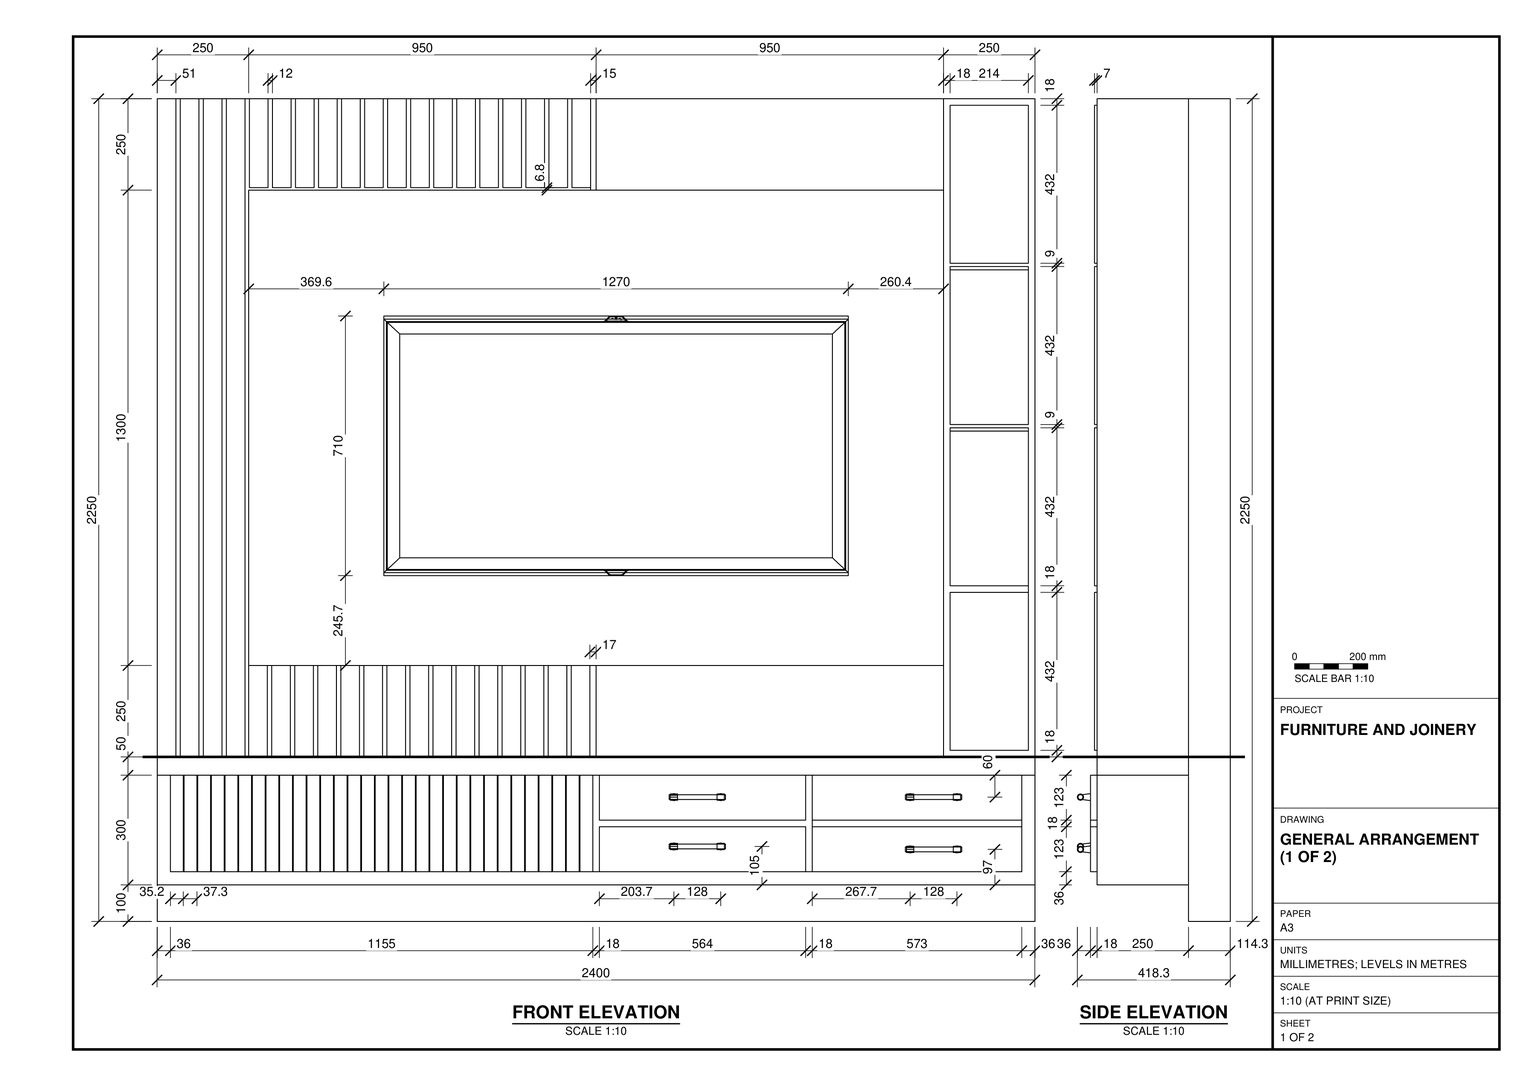
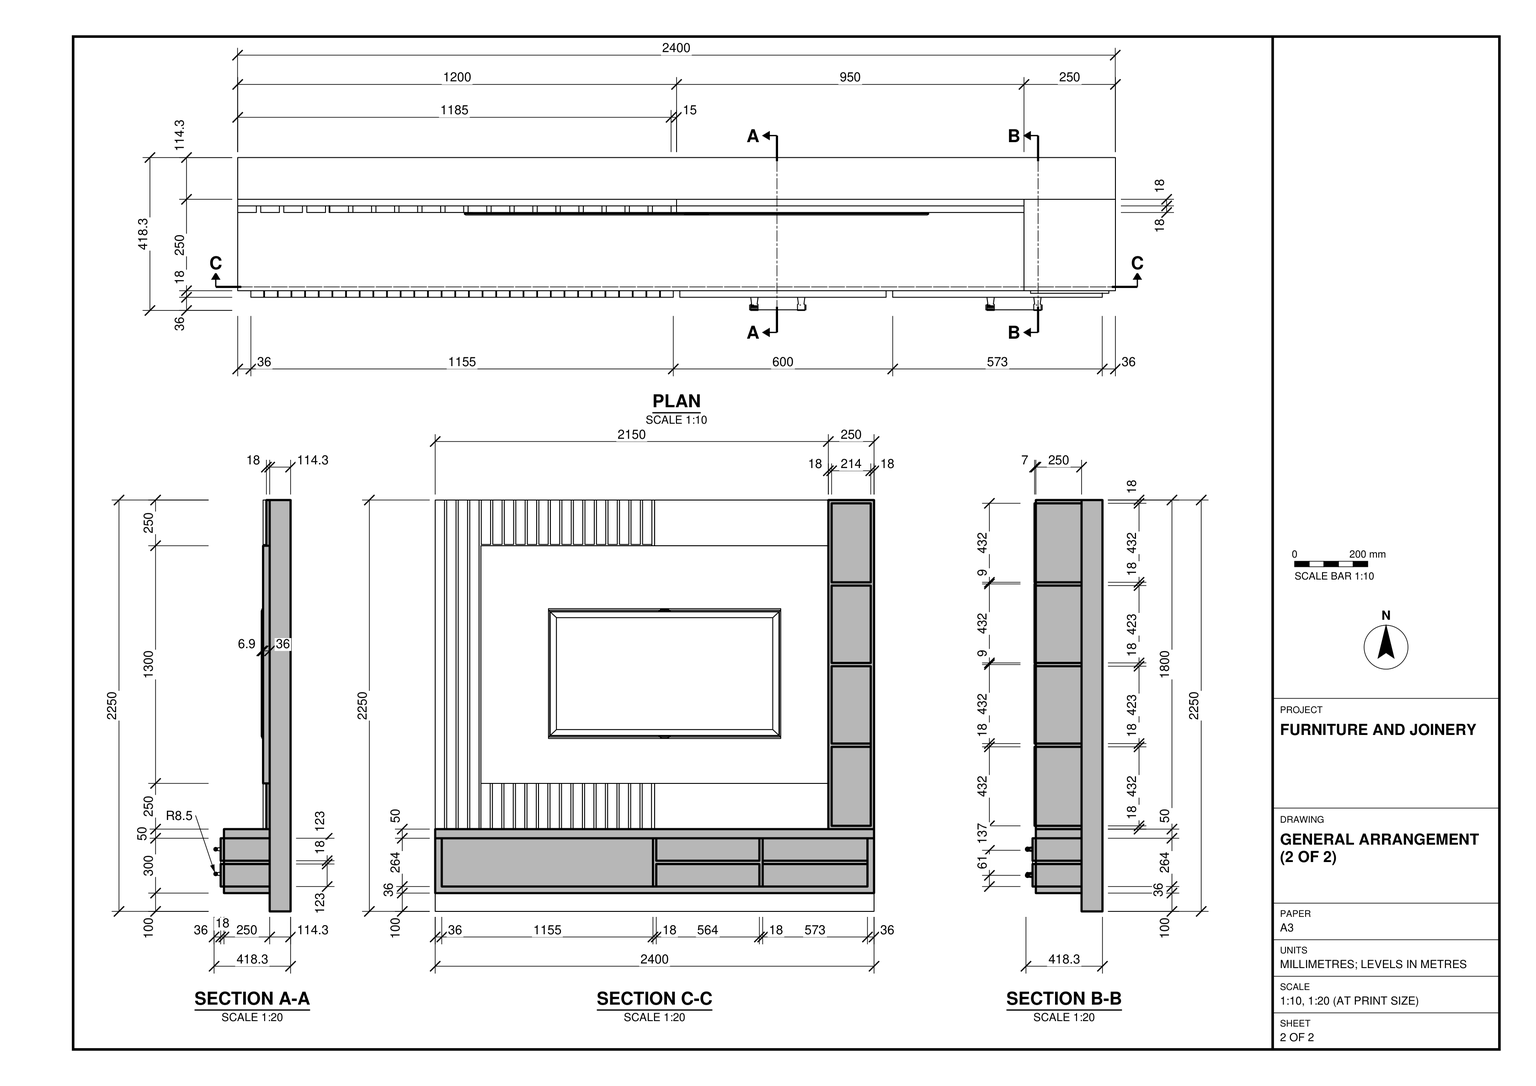
Build the media wall unit in SketchUp from task_files/diagram_01.pdf. Work in millimetres and use the floor line as the 0 mm datum. The complete unit is 2400 mm wide, 418.3 mm deep including the pulls, and 2250 mm high. Use the front elevation for the panel layout and the plan and sections for the depths of the backing, cabinet and projecting fronts.

Model the full-height backing and set the underside of the low cabinet 100 mm above the datum. Give the cabinet a continuous top, a broad vertically slatted front on the left and two banks of drawers on the right, with a horizontal pull on each drawer. Above the top, run the leftmost slats the full height of the upper assembly. Continue the slat pattern in shorter bands above and below the main display panel, leaving the right-hand portions of those bands plain. Position the framed display using the offset dimensions rather than centring it on the unit. Finish the right end with the narrow tower of four stacked compartments.

Keep the backing, cabinet, display surround and shelf tower as separate groups or components, and use components for repeated parts such as slats and pulls. Any decor or loose items may be suitable library components. Save one SketchUp model as output_files/media_wall_unit_with_slatted_panels_and_drawer_storage.skp.

# SketchUp Ruby script. Lengths in millimetres.
U = 1.mm
M = Sketchup.active_model
def pt(a) = Geom::Point3d.new(a.map { |v| v * U })
def face(e, loops, mat)
  f = e.add_face(loops[0].map { |a| pt(a) })
  loops[1..].each { |l| e.add_face(l.map { |a| pt(a) }).erase! }
  f.material = f.back_material = mat if mat
  f
end
# faces: each face lists its corners as indices into pts; further lists are holes
def faces(e, pts, list, mat = nil) = list.each { |f| face(e, (f[0].is_a?(Array) ? f : [f]).map { |l| l.map { |i| pts[i] } }, mat) }
# xy, xz, yz: faces in a plane at the given z, y or x. An outline is a flat list of corners, or four numbers for a rectangle; further outlines are holes
def ring(l) = l.size == 4 ? [[l[0], l[1]], [l[2], l[1]], [l[2], l[3]], [l[0], l[3]]] : l.each_slice(2).to_a
def flat(e, list, mat, &to3) = list.each { |f| face(e, (f[0].is_a?(Array) ? f : [f]).map { |l| ring(l).map { |u, v| to3.(u, v) } }, mat) }
def xy(e, z, list, mat = nil) = flat(e, list, mat) { |x, y| [x, y, z] }
def xz(e, y, list, mat = nil) = flat(e, list, mat) { |x, z| [x, y, z] }
def yz(e, x, list, mat = nil) = flat(e, list, mat) { |y, z| [x, y, z] }
def lines(e, pts, list) = list.each { |a, b| e.add_line(pt(pts[a]), pt(pts[b])) }
# prism: a flat outline (further loops are holes) pulled along v
def prism(e, loops, v, mat = nil)
  f = face(e, loops, mat); d = Geom::Vector3d.new(v.map { |x| x * U })
  f.pushpull(f.normal.samedirection?(d) ? d.length : -d.length)
end
def box(e, o, s, mat = nil) = prism(e, [[o, [o[0] + s[0], o[1], o[2]], [o[0] + s[0], o[1] + s[1], o[2]], [o[0], o[1] + s[1], o[2]]]], [0, 0, s[2]], mat)
def at(x, y, z, deg = 0) = Geom::Transformation.translation(pt([x, y, z])) * Geom::Transformation.rotation(ORIGIN, Z_AXIS, deg.degrees)
def axes(o, x, y, z) = Geom::Transformation.new([*x, 0, *y, 0, *z, 0, *pt(o).to_a, 1])
def part(name) = M.definitions.add(name)
# library, detail: a bought-in or finely detailed component or shape, given as its bounding box
def library(name, o, s) = part(name).tap { |d| box(d.entities, o, s) }
def detail(e, o, s) = box(e.add_group.entities, o, s)
def put(e, d, t, mat = nil) = e.add_instance(d, t).tap { |i| i.material = mat if mat }
def group(e, t, mat = nil) = e.add_group.tap { |g| g.transformation = t; g.material = mat if mat }.entities
root = M.entities
M.materials.add("0204 AP 9416 TWILIGHT PINK").color = [225, 165, 202]
M.materials.add("0466 AP 9679 Little Andaman-N").color = [89, 168, 184]
M.materials.add("Material__1").color = [190, 136, 85]
M.materials.add("Material__2").color = [51, 42, 44]
M.materials.add("Material__3").color = [119, 136, 107]
M.materials.add("[Marble Carrara Floor Tile]").color = [204, 208, 219]
M.materials.add("[Marble Carrara Gold Floor Tile]").color = [225, 223, 217]
M.materials.add("[Translucent Glass Blue]").color = [100, 149, 237]
M.materials["[Translucent Glass Blue]"].alpha = 0.5
M.materials.add("[Wood Cherry Original]").color = [152, 86, 42]
c1 = library("1-POIGNEE CLC2",[-77,-9.5,0],[154,19,36])
c2 = library("\#2",[-3043.7,-3043.7,2890.5],[6087.4,6087.4,441.9])
c3 = library("\#4",[-5204.9,-5393.6,-6012.5],[10776.8,6540.3,12002.4])
c4 = part("\#3")
put(c4.entities,c3,axes([-9.5,7866.8,0],[1.36765,0,0],[0,1.36765,0],[0,0,1.36765]),"Material__3")
c5 = library("\#1",[-4421.5,-4421.5,0],[8843,8843,3556])
c6 = part("9")
put(c6.entities,c2,at(-506.5,-626.4,0),"Material__2")
put(c6.entities,c4,axes([448.8,-828,1023.3],[0.29694,0.9549,0],[-0.21403,0.06656,0.97456],[0.9306,-0.28939,0.22414]))
put(c6.entities,c5,at(-506.5,-626.4,0),"Material__1")
c7 = library("Pots",[4666.4,-6982.1,0],[3244.2,3244.2,4850])
c8 = library("Television screen",[0,35.9,29],[912.5,6.9,513.2])
c9 = part("Group\#8")
box(c9.entities,[0,-18,0],[35.2,18,264])
c10 = part("Group20\#1")
xy(c10.entities,0,[[-600,-925,-549,925]])
xy(c10.entities,18,[[-600,-925,-549,925]])
xz(c10.entities,-925,[[-564,0,-549,18]])
xz(c10.entities,925,[[-600,0,-549,18]])
yz(c10.entities,-600,[[-925,0,925,18]])
yz(c10.entities,-549,[[-925,0,925,18]])
c11 = part("Group21\#1")
box(c11.entities,[-537,-925,0],[51,1850,18])
c12 = part("Group22\#1")
box(c12.entities,[-474,-925,0],[51,1850,18])
c13 = part("Group23\#1")
box(c13.entities,[-411,-925,0],[51,1850,18])
c14 = part("Group24\#1")
box(c14.entities,[-348,675,0],[51,250,18])
c15 = part("Group25\#1")
box(c15.entities,[-285,675,0],[51,250,18])
c16 = part("Group26\#1")
box(c16.entities,[-222,675,0],[51,250,18])
c17 = part("Group27\#1")
box(c17.entities,[-159,675,0],[51,250,18])
c18 = part("Group28\#1")
box(c18.entities,[-96,675,0],[51,250,18])
c19 = part("Group29\#1")
box(c19.entities,[-33,675,0],[51,250,18])
c20 = part("Group30\#1")
box(c20.entities,[30,675,0],[51,250,18])
c21 = part("Group31\#1")
box(c21.entities,[93,675,0],[51,250,18])
c22 = part("Group32\#1")
box(c22.entities,[156,675,0],[51,250,18])
c23 = part("Group33\#1")
box(c23.entities,[219,675,0],[51,250,18])
c24 = part("Group34\#1")
box(c24.entities,[282,675,0],[51,250,18])
c25 = part("Group35\#1")
box(c25.entities,[345,675,0],[51,250,18])
c26 = part("Group36\#1")
box(c26.entities,[408,675,0],[51,250,18])
c27 = part("Group37\#1")
box(c27.entities,[471,675,0],[51,250,18])
c28 = part("Group38\#1")
box(c28.entities,[534,675,0],[51,250,18])
c29 = part("Group18\#1")
put(c29.entities,c10,at(0,0,0))
put(c29.entities,c11,at(0,0,0))
put(c29.entities,c12,at(0,0,0))
put(c29.entities,c13,at(0,0,0))
put(c29.entities,c14,at(0,0,0))
put(c29.entities,c15,at(0,0,0))
put(c29.entities,c16,at(0,0,0))
put(c29.entities,c17,at(0,0,0))
put(c29.entities,c18,at(0,0,0))
put(c29.entities,c19,at(0,0,0))
put(c29.entities,c20,at(0,0,0))
put(c29.entities,c21,at(0,0,0))
put(c29.entities,c22,at(0,0,0))
put(c29.entities,c23,at(0,0,0))
put(c29.entities,c24,at(0,0,0))
put(c29.entities,c25,at(0,0,0))
put(c29.entities,c26,at(0,0,0))
put(c29.entities,c27,at(0,0,0))
put(c29.entities,c28,at(0,0,0))
c30 = part("Group41\#1")
box(c30.entities,[-475,-125,0],[51,250,18])
c31 = part("Group42\#1")
box(c31.entities,[-412,-125,0],[51,250,18])
c32 = part("Group43\#1")
box(c32.entities,[-349,-125,0],[51,250,18])
c33 = part("Group44\#1")
box(c33.entities,[-286,-125,0],[51,250,18])
c34 = part("Group45\#1")
box(c34.entities,[-223,-125,0],[51,250,18])
c35 = part("Group46\#1")
box(c35.entities,[-160,-125,0],[51,250,18])
c36 = part("Group47\#1")
box(c36.entities,[-97,-125,0],[51,250,18])
c37 = part("Group48\#1")
box(c37.entities,[-34,-125,0],[51,250,18])
c38 = part("Group49\#1")
box(c38.entities,[29,-125,0],[51,250,18])
c39 = part("Group50\#1")
box(c39.entities,[92,-125,0],[51,250,18])
c40 = part("Group51\#1")
box(c40.entities,[155,-125,0],[51,250,18])
c41 = part("Group52\#1")
box(c41.entities,[218,-125,0],[51,250,18])
c42 = part("Group53\#1")
box(c42.entities,[281,-125,0],[51,250,18])
c43 = part("Group54\#1")
box(c43.entities,[344,-125,0],[51,250,18])
c44 = part("Group55\#1")
box(c44.entities,[407,-125,0],[51,250,18])
c45 = part("Group39\#2")
put(c45.entities,c30,at(0,0,0))
put(c45.entities,c31,at(0,0,0))
put(c45.entities,c32,at(0,0,0))
put(c45.entities,c33,at(0,0,0))
put(c45.entities,c34,at(0,0,0))
put(c45.entities,c35,at(0,0,0))
put(c45.entities,c36,at(0,0,0))
put(c45.entities,c37,at(0,0,0))
put(c45.entities,c38,at(0,0,0))
put(c45.entities,c39,at(0,0,0))
put(c45.entities,c40,at(0,0,0))
put(c45.entities,c41,at(0,0,0))
put(c45.entities,c42,at(0,0,0))
put(c45.entities,c43,at(0,0,0))
put(c45.entities,c44,at(0,0,0))
xz(root,268,[[0,-100,2400,0]],"[Wood Cherry Original]")
put(root,c1,axes([1476.7,0,240],[1,0,0],[0,0,1],[0,-1,0]))
put(root,c1,axes([2122.7,0,240],[1,0,0],[0,0,1],[0,-1,0]))
put(root,c1,axes([1476.7,0,105],[1,0,0],[0,0,1],[0,-1,0]))
put(root,c1,axes([2122.7,0,97],[1,0,0],[0,0,1],[0,-1,0]))
put(root,c6,axes([2290,143.8,1709],[0.01076,0,0],[0,0.01262,0],[0,0,0.02626]))
put(root,c6,axes([2290,143.8,827],[0.01076,0,0],[0,0.01262,0],[0,0,0.02626]))
put(root,c7,axes([2110.8,308.3,1259],[0.02629,0,0],[0,0.02839,0],[0,0,0.0348]))
put(root,c7,axes([2100.2,297.2,368],[0.02629,0,0],[0,0.02839,0],[0,0,0.0348]))
put(root,c8,axes([619.6,189.2,805.6],[1.39179,0,0],[0,1,0],[0,0,1.38352]))
g1 = group(root,at(1209,18,177),"0466 AP 9679 Little Andaman-N")
box(g1,[0,-18,0],[564,18,123])
g2 = group(root,at(1209,18,36),"0204 AP 9416 TWILIGHT PINK")
box(g2,[0,-18,0],[564,18,123])
g3 = group(root,at(1800,18,177),"0204 AP 9416 TWILIGHT PINK")
box(g3,[-9,-18,0],[573,18,123])
g4 = group(root,at(1800,18,36),"0466 AP 9679 Little Andaman-N")
box(g4,[-9,-18,0],[573,18,123])
g5 = group(root,at(0,268,0),"[Wood Cherry Original]")
xy(g5,-100,[[0,0,2400,114.3]],"[Wood Cherry Original]")
xy(g5,2150,[[0,0,2400,114.3]],"[Wood Cherry Original]")
xz(g5,-18,[[1185,1900,1200,2150]])
xz(g5,0,[[1209,36,1773,159],[1791,36,2364,159],[1209,177,1773,300],[1791,177,2364,300],[2364,300,2400,350]])
xz(g5,0,[[2168,368,2382,800],[2168,818,2382,1241],[2168,1259,2382,1682],[2168,1700,2382,2132]],"[Wood Cherry Original]")
xz(g5,114.3,[[0,-100,2400,50],[0,50,2400,1268],[0,1268,2400,1709],[0,1709,2400,2150]],"[Wood Cherry Original]")
yz(g5,0,[[0,-100,114.3,2150]],"[Wood Cherry Original]")
yz(g5,2400,[[0,-100,114.3,2150]],"[Wood Cherry Original]")
p = [[250,0,350],[250,0,300]]
lines(g5,p,[[0,1]])
g6 = group(g5,at(36,0,36))
xz(g6,0,[[0,0,1155,264]])
g7 = group(g5,at(36,0,300),"[Wood Cherry Original]")
xy(g7,0,[[-36,-250,2364,0]])
xy(g7,50,[[-36,-250,2364,0]])
xz(g7,-250,[[-36,0,2364,50]])
xz(g7,0,[[-36,0,2364,50]])
yz(g7,-36,[[-250,0,0,50]])
yz(g7,2364,[[-250,0,0,50]])
g8 = group(g5,at(0,0,0),"[Wood Cherry Original]")
prism(g8,[[[36,0,300],[36,0,36],[1191,0,36],[1209,0,36],[1773,0,36],[1791,0,36],[2364,0,36],[2364,0,159],[2364,0,177],[2364,0,300],[2400,0,300],[2400,0,0],[0,0,0],[0,0,300]]],[0,-250,0])
g9 = group(g5,at(1191,0,36))
prism(g9,[[[18,0,141],[582,0,141],[582,0,264],[600,0,264],[600,0,141],[600,0,123],[600,0,0],[582,0,0],[582,0,123],[18,0,123],[18,0,0],[0,0,0],[0,0,123],[0,0,141],[0,0,264],[18,0,264]]],[0,-250,0])
g10 = group(g5,at(1791,0,159))
box(g10,[0,-250,0],[573,250,18])
g11 = group(g5,at(36,-250,36),"[Wood Cherry Original]")
xz(g11,0,[[35.2,0,1155,264]])
put(g11,c9,at(0,0,0))
put(g11,c9,at(37.3,0,0))
put(g11,c9,at(74.7,0,0))
put(g11,c9,at(112,0,0))
put(g11,c9,at(149.3,0,0))
put(g11,c9,at(186.6,0,0))
put(g11,c9,at(224,0,0))
put(g11,c9,at(261.3,0,0))
put(g11,c9,at(298.6,0,0))
put(g11,c9,at(335.9,0,0))
put(g11,c9,at(373.3,0,0))
put(g11,c9,at(410.6,0,0))
put(g11,c9,at(447.9,0,0))
put(g11,c9,at(485.3,0,0))
put(g11,c9,at(522.6,0,0))
put(g11,c9,at(559.9,0,0))
put(g11,c9,at(597.2,0,0))
put(g11,c9,at(634.6,0,0))
put(g11,c9,at(671.9,0,0))
put(g11,c9,at(709.2,0,0))
put(g11,c9,at(746.5,0,0))
put(g11,c9,at(783.9,0,0))
put(g11,c9,at(821.2,0,0))
put(g11,c9,at(858.5,0,0))
put(g11,c9,at(895.9,0,0))
put(g11,c9,at(933.2,0,0))
put(g11,c9,at(970.5,0,0))
put(g11,c9,at(1007.8,0,0))
put(g11,c9,at(1045.2,0,0))
put(g11,c9,at(1082.5,0,0))
put(g11,c9,at(1119.8,0,0))
g12 = group(g5,at(2150,0,350),"[Wood Cherry Original]")
xy(g12,0,[[0,-250,18,0],[18,-250,214,0],[214,-250,232,0],[232,-250,250,0]])
xy(g12,18,[[18,-250,214,0],[214,-250,232,0]])
xy(g12,450,[[18,-250,232,0]])
xy(g12,468,[[18,-250,232,0]])
xy(g12,891,[[18,-250,232,0]])
xy(g12,909,[[18,-250,232,0]])
xy(g12,1332,[[18,-250,232,0]])
xy(g12,1350,[[18,-250,232,0]])
xy(g12,1782,[[18,-250,232,0]])
xy(g12,1800,[[0,-250,250,0]])
xz(g12,-250,[[[0,0,250,1800],[18,18,18,450,232,450,232,468,18,468,18,891,232,891,232,18],[18,1350,232,1782],[18,909,232,1332]]])
xz(g12,0,[[[0,0,0,1782,18,1782,18,1350,232,1350,232,1782,250,1782,250,0],[18,18,232,18,232,891,18,891,18,468,232,468,232,450,18,450],[18,909,232,1332]],[0,1782,250,1800]])
yz(g12,0,[[-250,0,0,1800]])
yz(g12,18,[[-250,18,0,450],[-250,468,0,891],[-250,909,0,1332],[-250,1350,0,1414],[-250,1414,0,1782]])
yz(g12,232,[[-250,18,0,450],[-250,450,0,468],[-250,468,0,891],[-250,909,0,1332],[-250,1350,0,1782]])
yz(g12,250,[[-250,0,0,1800]])
g13 = group(g5,at(0,0,300),"[Wood Cherry Original]")
xy(g13,50,[[36,-18,250,0]])
xy(g13,1600,[[250,-18,1200,0]])
xy(g13,1850,[[0,-18,1200,0]])
xz(g13,0,[[36,0,0,50,0,1850,1200,1850,1200,1600,250,1600,250,50,36,50]])
yz(g13,0,[[-18,50,0,1850]])
yz(g13,36,[[-18,0,0,50]])
yz(g13,250,[[-18,50,0,1600]])
yz(g13,1200,[[-18,1600,0,1850]])
p = [[0,0,50],[36,0,0],[36,-18,0],[0,-18,50]]
faces(g13,p,[[0,1,2,3]])
put(g13,c29,axes([600,-18,950],[1,0,0],[0,0,0.97297],[0,-1,0]))
g14 = group(g5,at(1200,0,1900))
xy(g14,0,[[0,-18,950,0]],"[Marble Carrara Gold Floor Tile]")
xy(g14,250,[[0,-18,950,0]],"[Marble Carrara Gold Floor Tile]")
xz(g14,-18,[[0,0,950,250]])
xz(g14,0,[[0,0,950,250]],"[Marble Carrara Gold Floor Tile]")
yz(g14,0,[[-18,0,0,250]],"[Marble Carrara Gold Floor Tile]")
yz(g14,950,[[-18,0,0,250]],"[Marble Carrara Gold Floor Tile]")
g15 = group(g5,at(250,0,350),"[Wood Cherry Original]")
xy(g15,0,[[0,-18,941,0],[941,-18,950,0]])
xy(g15,250,[[0,-18,950,0]])
xz(g15,0,[[0,0,950,250]])
yz(g15,0,[[-18,0,0,250]])
yz(g15,950,[[-18,0,0,250]])
put(g15,c45,axes([475,-18,125],[1,0,0],[0,0,1],[0,-1,0]))
g16 = group(g5,at(1200,0,350))
prism(g16,[[[0,0,250],[950,0,250],[950,0,0],[591,0,0],[573,0,0],[9,0,0],[0,0,0]]],[0,-18,0])
g17 = group(g5,at(250,0,600),"0466 AP 9679 Little Andaman-N")
xy(g17,0,[[0,-36,950,0],[950,-36,1900,0]],"[Marble Carrara Floor Tile]")
xy(g17,1300,[[0,-36,950,0],[950,-36,1900,0]],"[Marble Carrara Floor Tile]")
xz(g17,-36,[[0,0,1900,1300]])
xz(g17,0,[[0,0,1900,1300]],"[Marble Carrara Floor Tile]")
yz(g17,0,[[-36,0,0,1300]],"[Marble Carrara Floor Tile]")
yz(g17,1900,[[-36,0,0,1300]],"[Marble Carrara Floor Tile]")
g18 = group(g17,at(369.6,-36,245.7))
xz(g18,0,[[0,0,1270,710]])
g19 = group(root,at(2168,18,1700),"[Translucent Glass Blue]")
box(g19,[0,-7,0],[214,7,432])
g20 = group(root,at(2168,18,1259),"[Translucent Glass Blue]")
box(g20,[0,-7,0],[214,7,432])
g21 = group(root,at(2168,18,818),"[Translucent Glass Blue]")
box(g21,[0,-7,0],[214,7,432])
g22 = group(root,at(2168,18,368),"[Translucent Glass Blue]")
box(g22,[0,-7,0],[214,7,432])
